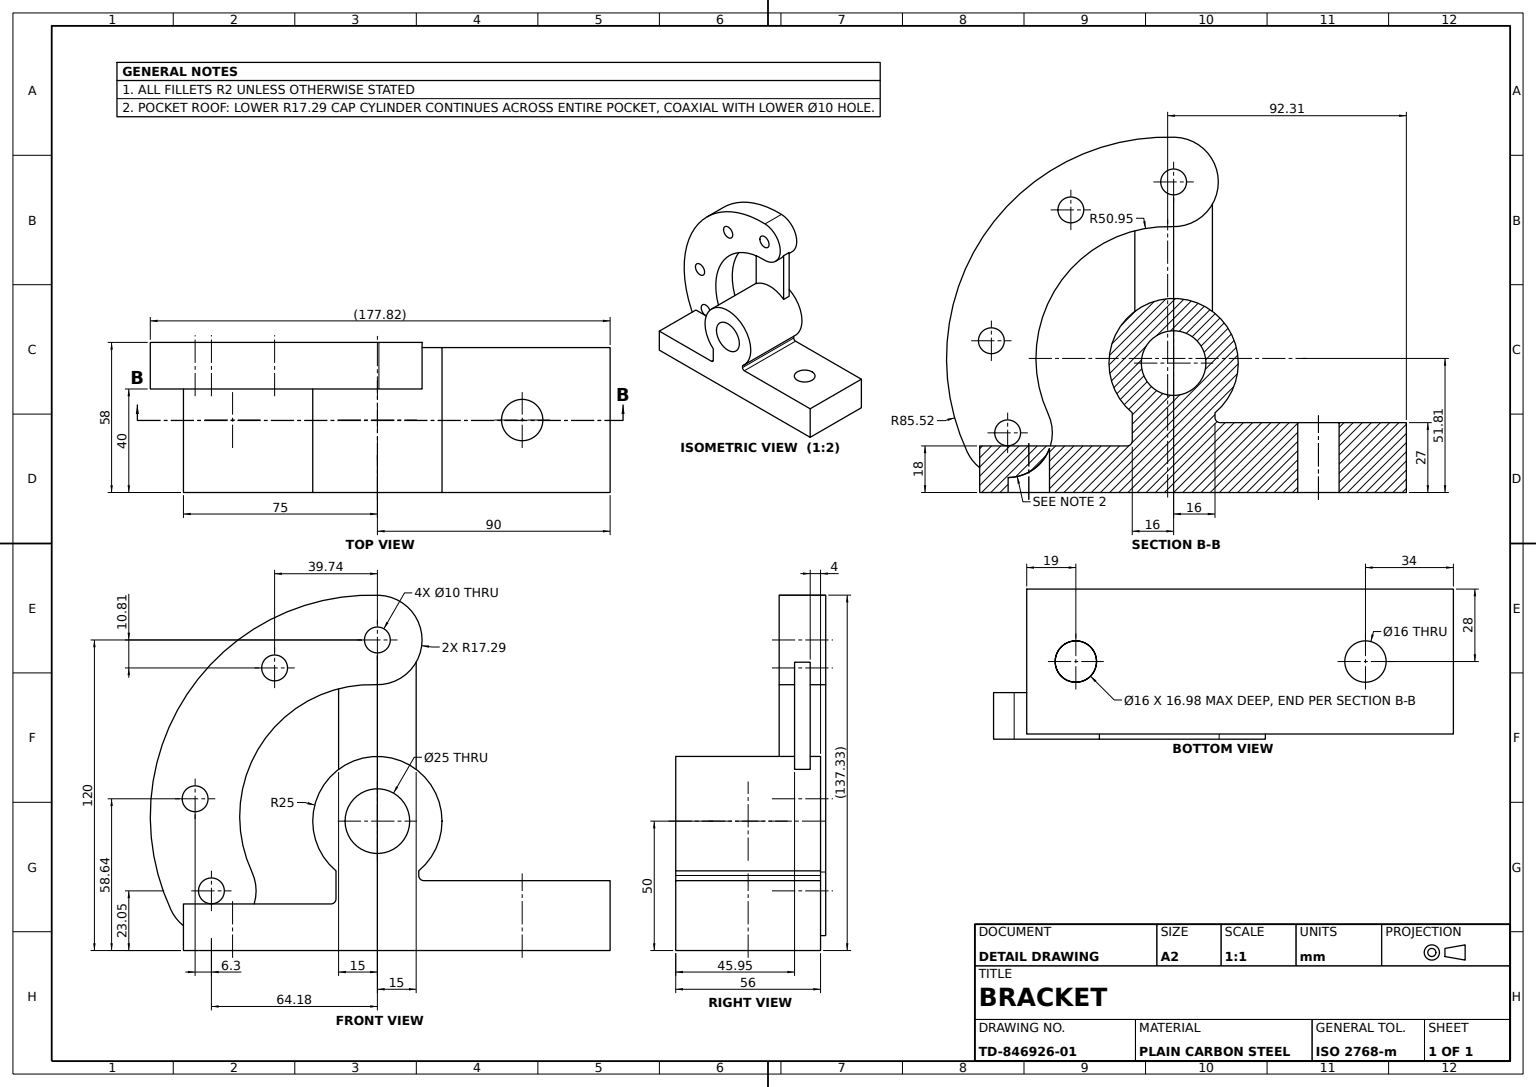
ISO-10303-21;
HEADER;
FILE_DESCRIPTION((''),'2;1');
FILE_NAME('','',(''),(''),'','','');
FILE_SCHEMA(('AUTOMOTIVE_DESIGN'));
ENDSEC;
DATA;
#1=APPLICATION_CONTEXT('');
#2=PRODUCT_CONTEXT('',#1,'mechanical');
#3=PRODUCT('','','',(#2));
#4=PRODUCT_DEFINITION_FORMATION('','',#3);
#5=PRODUCT_DEFINITION_CONTEXT('',#1,'design');
#6=PRODUCT_DEFINITION('','',#4,#5);
#7=PRODUCT_DEFINITION_SHAPE('','',#6);
#8=(LENGTH_UNIT()NAMED_UNIT(*)SI_UNIT(.MILLI.,.METRE.));
#9=(NAMED_UNIT(*)PLANE_ANGLE_UNIT()SI_UNIT($,.RADIAN.));
#10=(NAMED_UNIT(*)SI_UNIT($,.STERADIAN.)SOLID_ANGLE_UNIT());
#11=UNCERTAINTY_MEASURE_WITH_UNIT(LENGTH_MEASURE(1.E-05),#8,'distance_accuracy_value','');
#12=(GEOMETRIC_REPRESENTATION_CONTEXT(3)GLOBAL_UNCERTAINTY_ASSIGNED_CONTEXT((#11))GLOBAL_UNIT_ASSIGNED_CONTEXT((#8,#9,#10))REPRESENTATION_CONTEXT('',''));
#13=CARTESIAN_POINT('',(-5.,120.,-40.));
#14=VERTEX_POINT('',#13);
#15=CARTESIAN_POINT('',(-5.,120.,-58.));
#16=VERTEX_POINT('',#15);
#17=CARTESIAN_POINT('',(-5.,120.,-18.));
#18=DIRECTION('',(0.,0.,-1.));
#19=VECTOR('',#18,1000.);
#20=LINE('',#17,#19);
#21=EDGE_CURVE('',#14,#16,#20,.T.);
#22=ORIENTED_EDGE('',*,*,#21,.T.);
#23=CARTESIAN_POINT('',(5.,120.,-58.));
#24=VERTEX_POINT('',#23);
#25=CARTESIAN_POINT('',(0.,120.,-58.));
#26=DIRECTION('',(-1.,0.,0.));
#27=AXIS2_PLACEMENT_3D('',#25,#18,#26);
#28=CIRCLE('',#27,5.);
#29=EDGE_CURVE('',#16,#24,#28,.T.);
#30=ORIENTED_EDGE('',*,*,#29,.T.);
#31=CARTESIAN_POINT('',(5.,120.,-40.));
#32=VERTEX_POINT('',#31);
#33=CARTESIAN_POINT('',(5.,120.,-18.));
#34=LINE('',#33,#19);
#35=EDGE_CURVE('',#32,#24,#34,.T.);
#36=ORIENTED_EDGE('',*,*,#35,.F.);
#37=CARTESIAN_POINT('',(0.,120.,-40.));
#38=DIRECTION('',(0.,0.,1.));
#39=DIRECTION('',(1.,0.,0.));
#40=AXIS2_PLACEMENT_3D('',#37,#38,#39);
#41=CIRCLE('',#40,5.);
#42=EDGE_CURVE('',#32,#14,#41,.T.);
#43=ORIENTED_EDGE('',*,*,#42,.T.);
#44=EDGE_LOOP('',(#22,#30,#36,#43));
#45=FACE_OUTER_BOUND('',#44,.T.);
#46=CARTESIAN_POINT('',(0.,120.,-18.));
#47=AXIS2_PLACEMENT_3D('',#46,#18,#26);
#48=CYLINDRICAL_SURFACE('',#47,5.);
#49=ADVANCED_FACE('',(#45),#48,.F.);
#50=CARTESIAN_POINT('',(-12.5,50.,-56.));
#51=VERTEX_POINT('',#50);
#52=CARTESIAN_POINT('',(-12.5,50.,0.));
#53=VERTEX_POINT('',#52);
#54=VECTOR('',#38,1000.);
#55=LINE('',#50,#54);
#56=EDGE_CURVE('',#51,#53,#55,.T.);
#57=ORIENTED_EDGE('',*,*,#56,.T.);
#58=CARTESIAN_POINT('',(12.5,50.,0.));
#59=VERTEX_POINT('',#58);
#60=CARTESIAN_POINT('',(0.,50.,0.));
#61=AXIS2_PLACEMENT_3D('',#60,#38,#39);
#62=CIRCLE('',#61,12.5);
#63=EDGE_CURVE('',#53,#59,#62,.T.);
#64=ORIENTED_EDGE('',*,*,#63,.T.);
#65=CARTESIAN_POINT('',(12.5,50.,-56.));
#66=VERTEX_POINT('',#65);
#67=LINE('',#65,#54);
#68=EDGE_CURVE('',#66,#59,#67,.T.);
#69=ORIENTED_EDGE('',*,*,#68,.F.);
#70=CARTESIAN_POINT('',(0.,50.,-56.));
#71=AXIS2_PLACEMENT_3D('',#70,#38,#39);
#72=CIRCLE('',#71,12.5);
#73=EDGE_CURVE('',#51,#66,#72,.T.);
#74=ORIENTED_EDGE('',*,*,#73,.F.);
#75=EDGE_LOOP('',(#57,#64,#69,#74));
#76=FACE_OUTER_BOUND('',#75,.T.);
#77=CYLINDRICAL_SURFACE('',#71,12.5);
#78=ADVANCED_FACE('',(#76),#77,.F.);
#79=CARTESIAN_POINT('',(-69.182521,23.053551,-40.));
#80=VERTEX_POINT('',#79);
#81=CARTESIAN_POINT('',(-59.182521,23.053551,-40.));
#82=VERTEX_POINT('',#81);
#83=CARTESIAN_POINT('',(-64.182521,23.053551,-40.));
#84=AXIS2_PLACEMENT_3D('',#83,#38,#39);
#85=CIRCLE('',#84,5.);
#86=EDGE_CURVE('',#80,#82,#85,.T.);
#87=ORIENTED_EDGE('',*,*,#86,.T.);
#88=CARTESIAN_POINT('',(-59.182521,23.053551,-58.));
#89=VERTEX_POINT('',#88);
#90=CARTESIAN_POINT('',(-59.182521,23.053551,-18.));
#91=LINE('',#90,#19);
#92=EDGE_CURVE('',#82,#89,#91,.T.);
#93=ORIENTED_EDGE('',*,*,#92,.T.);
#94=CARTESIAN_POINT('',(-69.182521,23.053551,-58.));
#95=VERTEX_POINT('',#94);
#96=CARTESIAN_POINT('',(-64.182521,23.053551,-58.));
#97=AXIS2_PLACEMENT_3D('',#96,#18,#26);
#98=CIRCLE('',#97,5.);
#99=EDGE_CURVE('',#89,#95,#98,.T.);
#100=ORIENTED_EDGE('',*,*,#99,.T.);
#101=CARTESIAN_POINT('',(-69.182521,23.053551,-18.));
#102=LINE('',#101,#19);
#103=EDGE_CURVE('',#80,#95,#102,.T.);
#104=ORIENTED_EDGE('',*,*,#103,.F.);
#105=EDGE_LOOP('',(#87,#93,#100,#104));
#106=FACE_OUTER_BOUND('',#105,.T.);
#107=CARTESIAN_POINT('',(-64.182521,23.053551,-18.));
#108=AXIS2_PLACEMENT_3D('',#107,#18,#26);
#109=CYLINDRICAL_SURFACE('',#108,5.);
#110=ADVANCED_FACE('',(#106),#109,.F.);
#111=CARTESIAN_POINT('',(15.,111.408742,-45.952641));
#112=VERTEX_POINT('',#111);
#113=CARTESIAN_POINT('',(15.,111.408742,-52.));
#114=VERTEX_POINT('',#113);
#115=CARTESIAN_POINT('',(15.,111.408742,-58.));
#116=LINE('',#115,#19);
#117=EDGE_CURVE('',#112,#114,#116,.T.);
#118=ORIENTED_EDGE('',*,*,#117,.F.);
#119=CARTESIAN_POINT('',(15.,70.,-45.952641));
#120=VERTEX_POINT('',#119);
#121=CARTESIAN_POINT('',(15.,-0.001,-45.952641));
#122=DIRECTION('',(0.,1.,0.));
#123=VECTOR('',#122,1000.);
#124=LINE('',#121,#123);
#125=EDGE_CURVE('',#120,#112,#124,.T.);
#126=ORIENTED_EDGE('',*,*,#125,.F.);
#127=CARTESIAN_POINT('',(15.,70.,-52.));
#128=VERTEX_POINT('',#127);
#129=CARTESIAN_POINT('',(15.,70.,-56.));
#130=LINE('',#129,#19);
#131=EDGE_CURVE('',#120,#128,#130,.T.);
#132=ORIENTED_EDGE('',*,*,#131,.T.);
#133=CARTESIAN_POINT('',(15.,65.595641,-52.));
#134=LINE('',#133,#123);
#135=EDGE_CURVE('',#128,#114,#134,.T.);
#136=ORIENTED_EDGE('',*,*,#135,.T.);
#137=EDGE_LOOP('',(#118,#126,#132,#136));
#138=FACE_OUTER_BOUND('',#137,.T.);
#139=CARTESIAN_POINT('',(15.,65.595641,-118.127564));
#140=AXIS2_PLACEMENT_3D('',#139,#39,#18);
#141=PLANE('',#140);
#142=ADVANCED_FACE('',(#138),#141,.T.);
#143=CARTESIAN_POINT('',(56.,0.,-20.));
#144=VERTEX_POINT('',#143);
#145=CARTESIAN_POINT('',(56.,0.,-36.));
#146=VERTEX_POINT('',#145);
#147=CARTESIAN_POINT('',(56.,0.,-28.));
#148=AXIS2_PLACEMENT_3D('',#147,#122,#38);
#149=CIRCLE('',#148,8.);
#150=EDGE_CURVE('',#144,#146,#149,.T.);
#151=ORIENTED_EDGE('',*,*,#150,.T.);
#152=EDGE_CURVE('',#146,#144,#149,.T.);
#153=ORIENTED_EDGE('',*,*,#152,.T.);
#154=EDGE_LOOP('',(#151,#153));
#155=FACE_BOUND('',#154,.T.);
#156=CARTESIAN_POINT('',(-56.,0.,-20.));
#157=VERTEX_POINT('',#156);
#158=CARTESIAN_POINT('',(-56.,0.,-36.));
#159=VERTEX_POINT('',#158);
#160=CARTESIAN_POINT('',(-56.,0.,-28.));
#161=AXIS2_PLACEMENT_3D('',#160,#122,#18);
#162=CIRCLE('',#161,8.);
#163=EDGE_CURVE('',#157,#159,#162,.T.);
#164=ORIENTED_EDGE('',*,*,#163,.T.);
#165=EDGE_CURVE('',#159,#157,#162,.T.);
#166=ORIENTED_EDGE('',*,*,#165,.T.);
#167=EDGE_LOOP('',(#164,#166));
#168=FACE_BOUND('',#167,.T.);
#169=CARTESIAN_POINT('',(90.,0.,-56.));
#170=VERTEX_POINT('',#169);
#171=CARTESIAN_POINT('',(90.,0.,0.));
#172=VERTEX_POINT('',#171);
#173=LINE('',#169,#54);
#174=EDGE_CURVE('',#170,#172,#173,.T.);
#175=ORIENTED_EDGE('',*,*,#174,.T.);
#176=CARTESIAN_POINT('',(-75.,0.,0.));
#177=VERTEX_POINT('',#176);
#178=CARTESIAN_POINT('',(0.,0.,0.));
#179=VECTOR('',#39,1000.);
#180=LINE('',#178,#179);
#181=EDGE_CURVE('',#177,#172,#180,.T.);
#182=ORIENTED_EDGE('',*,*,#181,.F.);
#183=CARTESIAN_POINT('',(-75.,0.,-56.));
#184=VERTEX_POINT('',#183);
#185=LINE('',#183,#54);
#186=EDGE_CURVE('',#184,#177,#185,.T.);
#187=ORIENTED_EDGE('',*,*,#186,.F.);
#188=LINE('',#169,#179);
#189=EDGE_CURVE('',#184,#170,#188,.T.);
#190=ORIENTED_EDGE('',*,*,#189,.T.);
#191=EDGE_LOOP('',(#175,#182,#187,#190));
#192=FACE_OUTER_BOUND('',#191,.T.);
#193=CARTESIAN_POINT('',(0.,0.,-56.));
#194=DIRECTION('',(0.,-1.,0.));
#195=AXIS2_PLACEMENT_3D('',#193,#194,#18);
#196=PLANE('',#195);
#197=ADVANCED_FACE('',(#155,#168,#192),#196,.T.);
#198=CARTESIAN_POINT('',(56.,27.,-36.));
#199=VERTEX_POINT('',#198);
#200=LINE('',#145,#123);
#201=EDGE_CURVE('',#146,#199,#200,.T.);
#202=ORIENTED_EDGE('',*,*,#201,.T.);
#203=CARTESIAN_POINT('',(56.,27.,-20.));
#204=VERTEX_POINT('',#203);
#205=CARTESIAN_POINT('',(56.,27.,-28.));
#206=AXIS2_PLACEMENT_3D('',#205,#122,#38);
#207=CIRCLE('',#206,8.);
#208=EDGE_CURVE('',#199,#204,#207,.T.);
#209=ORIENTED_EDGE('',*,*,#208,.T.);
#210=LINE('',#143,#123);
#211=EDGE_CURVE('',#144,#204,#210,.T.);
#212=ORIENTED_EDGE('',*,*,#211,.F.);
#213=ORIENTED_EDGE('',*,*,#152,.F.);
#214=EDGE_LOOP('',(#202,#209,#212,#213));
#215=FACE_OUTER_BOUND('',#214,.T.);
#216=CYLINDRICAL_SURFACE('',#148,8.);
#217=ADVANCED_FACE('',(#215),#216,.F.);
#218=CARTESIAN_POINT('',(-16.,30.790627,-56.));
#219=VERTEX_POINT('',#218);
#220=CARTESIAN_POINT('',(-16.,20.,-56.));
#221=VERTEX_POINT('',#220);
#222=VECTOR('',#194,1000.);
#223=LINE('',#218,#222);
#224=EDGE_CURVE('',#219,#221,#223,.T.);
#225=ORIENTED_EDGE('',*,*,#224,.T.);
#226=CARTESIAN_POINT('',(-16.,20.,0.));
#227=VERTEX_POINT('',#226);
#228=LINE('',#226,#54);
#229=EDGE_CURVE('',#221,#227,#228,.T.);
#230=ORIENTED_EDGE('',*,*,#229,.T.);
#231=CARTESIAN_POINT('',(-16.,30.790627,0.));
#232=VERTEX_POINT('',#231);
#233=LINE('',#231,#222);
#234=EDGE_CURVE('',#232,#227,#233,.T.);
#235=ORIENTED_EDGE('',*,*,#234,.F.);
#236=LINE('',#218,#54);
#237=EDGE_CURVE('',#219,#232,#236,.T.);
#238=ORIENTED_EDGE('',*,*,#237,.F.);
#239=EDGE_LOOP('',(#225,#230,#235,#238));
#240=FACE_OUTER_BOUND('',#239,.T.);
#241=AXIS2_PLACEMENT_3D('',#218,#26,#194);
#242=PLANE('',#241);
#243=ADVANCED_FACE('',(#240),#242,.T.);
#244=CARTESIAN_POINT('',(-25.,50.,-56.));
#245=VERTEX_POINT('',#244);
#246=CARTESIAN_POINT('',(-25.,50.,0.));
#247=VERTEX_POINT('',#246);
#248=LINE('',#244,#54);
#249=EDGE_CURVE('',#245,#247,#248,.T.);
#250=ORIENTED_EDGE('',*,*,#249,.F.);
#251=CIRCLE('',#71,25.);
#252=EDGE_CURVE('',#245,#219,#251,.T.);
#253=ORIENTED_EDGE('',*,*,#252,.T.);
#254=ORIENTED_EDGE('',*,*,#237,.T.);
#255=CIRCLE('',#61,25.);
#256=EDGE_CURVE('',#247,#232,#255,.T.);
#257=ORIENTED_EDGE('',*,*,#256,.F.);
#258=EDGE_LOOP('',(#250,#253,#254,#257));
#259=FACE_OUTER_BOUND('',#258,.T.);
#260=CYLINDRICAL_SURFACE('',#71,25.);
#261=ADVANCED_FACE('',(#259),#260,.T.);
#262=ORIENTED_EDGE('',*,*,#63,.F.);
#263=EDGE_CURVE('',#59,#53,#62,.T.);
#264=ORIENTED_EDGE('',*,*,#263,.F.);
#265=EDGE_LOOP('',(#262,#264));
#266=FACE_BOUND('',#265,.T.);
#267=CARTESIAN_POINT('',(90.,27.,0.));
#268=VERTEX_POINT('',#267);
#269=CARTESIAN_POINT('',(18.,27.,0.));
#270=VERTEX_POINT('',#269);
#271=CARTESIAN_POINT('',(0.,27.,0.));
#272=VECTOR('',#26,1000.);
#273=LINE('',#271,#272);
#274=EDGE_CURVE('',#268,#270,#273,.T.);
#275=ORIENTED_EDGE('',*,*,#274,.T.);
#276=CARTESIAN_POINT('',(16.,29.,0.));
#277=VERTEX_POINT('',#276);
#278=CARTESIAN_POINT('',(18.,29.,0.));
#279=AXIS2_PLACEMENT_3D('',#278,#18,#26);
#280=CIRCLE('',#279,2.);
#281=EDGE_CURVE('',#270,#277,#280,.T.);
#282=ORIENTED_EDGE('',*,*,#281,.T.);
#283=CARTESIAN_POINT('',(16.,30.790627,0.));
#284=VERTEX_POINT('',#283);
#285=LINE('',#283,#123);
#286=EDGE_CURVE('',#277,#284,#285,.T.);
#287=ORIENTED_EDGE('',*,*,#286,.T.);
#288=CARTESIAN_POINT('',(25.,50.,0.));
#289=VERTEX_POINT('',#288);
#290=EDGE_CURVE('',#284,#289,#255,.T.);
#291=ORIENTED_EDGE('',*,*,#290,.T.);
#292=EDGE_CURVE('',#289,#247,#255,.T.);
#293=ORIENTED_EDGE('',*,*,#292,.T.);
#294=ORIENTED_EDGE('',*,*,#256,.T.);
#295=ORIENTED_EDGE('',*,*,#234,.T.);
#296=CARTESIAN_POINT('',(-18.,18.,0.));
#297=VERTEX_POINT('',#296);
#298=CARTESIAN_POINT('',(-18.,20.,0.));
#299=AXIS2_PLACEMENT_3D('',#298,#18,#26);
#300=CIRCLE('',#299,2.);
#301=EDGE_CURVE('',#227,#297,#300,.T.);
#302=ORIENTED_EDGE('',*,*,#301,.T.);
#303=CARTESIAN_POINT('',(-75.,18.,0.));
#304=VERTEX_POINT('',#303);
#305=LINE('',#303,#272);
#306=EDGE_CURVE('',#297,#304,#305,.T.);
#307=ORIENTED_EDGE('',*,*,#306,.T.);
#308=LINE('',#176,#222);
#309=EDGE_CURVE('',#304,#177,#308,.T.);
#310=ORIENTED_EDGE('',*,*,#309,.T.);
#311=ORIENTED_EDGE('',*,*,#181,.T.);
#312=LINE('',#267,#123);
#313=EDGE_CURVE('',#172,#268,#312,.T.);
#314=ORIENTED_EDGE('',*,*,#313,.T.);
#315=EDGE_LOOP('',(#275,#282,#287,#291,#293,#294,#295,#302,#307,#310,#311,#314));
#316=FACE_OUTER_BOUND('',#315,.T.);
#317=AXIS2_PLACEMENT_3D('',#178,#18,#26);
#318=PLANE('',#317);
#319=ADVANCED_FACE('',(#266,#316),#318,.F.);
#320=ORIENTED_EDGE('',*,*,#286,.F.);
#321=CARTESIAN_POINT('',(16.,29.,-56.));
#322=VERTEX_POINT('',#321);
#323=LINE('',#321,#19);
#324=EDGE_CURVE('',#277,#322,#323,.T.);
#325=ORIENTED_EDGE('',*,*,#324,.T.);
#326=CARTESIAN_POINT('',(16.,30.790627,-56.));
#327=VERTEX_POINT('',#326);
#328=LINE('',#326,#123);
#329=EDGE_CURVE('',#322,#327,#328,.T.);
#330=ORIENTED_EDGE('',*,*,#329,.T.);
#331=LINE('',#326,#54);
#332=EDGE_CURVE('',#327,#284,#331,.T.);
#333=ORIENTED_EDGE('',*,*,#332,.T.);
#334=EDGE_LOOP('',(#320,#325,#330,#333));
#335=FACE_OUTER_BOUND('',#334,.T.);
#336=AXIS2_PLACEMENT_3D('',#326,#39,#122);
#337=PLANE('',#336);
#338=ADVANCED_FACE('',(#335),#337,.T.);
#339=ORIENTED_EDGE('',*,*,#281,.F.);
#340=CARTESIAN_POINT('',(18.,27.,-56.));
#341=VERTEX_POINT('',#340);
#342=LINE('',#269,#54);
#343=EDGE_CURVE('',#341,#270,#342,.T.);
#344=ORIENTED_EDGE('',*,*,#343,.F.);
#345=CARTESIAN_POINT('',(18.,29.,-56.));
#346=AXIS2_PLACEMENT_3D('',#345,#38,#26);
#347=CIRCLE('',#346,2.);
#348=EDGE_CURVE('',#322,#341,#347,.T.);
#349=ORIENTED_EDGE('',*,*,#348,.F.);
#350=ORIENTED_EDGE('',*,*,#324,.F.);
#351=EDGE_LOOP('',(#339,#344,#349,#350));
#352=FACE_OUTER_BOUND('',#351,.T.);
#353=AXIS2_PLACEMENT_3D('',#345,#38,#39);
#354=CYLINDRICAL_SURFACE('',#353,2.);
#355=ADVANCED_FACE('',(#352),#354,.F.);
#356=CARTESIAN_POINT('',(-79.858671,15.768771,-58.));
#357=VERTEX_POINT('',#356);
#358=CARTESIAN_POINT('',(-79.858671,15.768771,-40.));
#359=VERTEX_POINT('',#358);
#360=LINE('',#356,#54);
#361=EDGE_CURVE('',#357,#359,#360,.T.);
#362=ORIENTED_EDGE('',*,*,#361,.F.);
#363=CARTESIAN_POINT('',(-46.896408,23.053551,-58.));
#364=VERTEX_POINT('',#363);
#365=AXIS2_PLACEMENT_3D('',#96,#38,#39);
#366=CIRCLE('',#365,17.286113);
#367=EDGE_CURVE('',#357,#364,#366,.T.);
#368=ORIENTED_EDGE('',*,*,#367,.T.);
#369=CARTESIAN_POINT('',(-46.896408,23.053551,-40.));
#370=VERTEX_POINT('',#369);
#371=LINE('',#363,#54);
#372=EDGE_CURVE('',#364,#370,#371,.T.);
#373=ORIENTED_EDGE('',*,*,#372,.T.);
#374=CARTESIAN_POINT('',(-47.651601,18.,-40.));
#375=VERTEX_POINT('',#374);
#376=CIRCLE('',#84,17.286113);
#377=EDGE_CURVE('',#375,#370,#376,.T.);
#378=ORIENTED_EDGE('',*,*,#377,.F.);
#379=CARTESIAN_POINT('',(-47.651601,18.,-56.));
#380=VERTEX_POINT('',#379);
#381=CARTESIAN_POINT('',(-47.651601,18.,-58.));
#382=LINE('',#381,#19);
#383=EDGE_CURVE('',#375,#380,#382,.T.);
#384=ORIENTED_EDGE('',*,*,#383,.T.);
#385=CARTESIAN_POINT('',(-75.,9.57053,-56.));
#386=VERTEX_POINT('',#385);
#387=CARTESIAN_POINT('',(-64.182521,23.053551,-56.));
#388=AXIS2_PLACEMENT_3D('',#387,#18,#26);
#389=CIRCLE('',#388,17.286113);
#390=EDGE_CURVE('',#380,#386,#389,.T.);
#391=ORIENTED_EDGE('',*,*,#390,.T.);
#392=CARTESIAN_POINT('',(-75.,9.57053,-40.));
#393=VERTEX_POINT('',#392);
#394=CARTESIAN_POINT('',(-75.,9.57053,-58.));
#395=LINE('',#394,#54);
#396=EDGE_CURVE('',#386,#393,#395,.T.);
#397=ORIENTED_EDGE('',*,*,#396,.T.);
#398=EDGE_CURVE('',#359,#393,#376,.T.);
#399=ORIENTED_EDGE('',*,*,#398,.F.);
#400=EDGE_LOOP('',(#362,#368,#373,#378,#384,#391,#397,#399));
#401=FACE_OUTER_BOUND('',#400,.T.);
#402=CYLINDRICAL_SURFACE('',#365,17.286113);
#403=ADVANCED_FACE('',(#401),#402,.T.);
#404=CARTESIAN_POINT('',(-75.482391,58.635503,-40.));
#405=VERTEX_POINT('',#404);
#406=CARTESIAN_POINT('',(-75.482391,58.635503,-58.));
#407=VERTEX_POINT('',#406);
#408=CARTESIAN_POINT('',(-75.482391,58.635503,-18.));
#409=LINE('',#408,#19);
#410=EDGE_CURVE('',#405,#407,#409,.T.);
#411=ORIENTED_EDGE('',*,*,#410,.F.);
#412=CARTESIAN_POINT('',(-65.482391,58.635503,-40.));
#413=VERTEX_POINT('',#412);
#414=CARTESIAN_POINT('',(-70.482391,58.635503,-40.));
#415=AXIS2_PLACEMENT_3D('',#414,#38,#39);
#416=CIRCLE('',#415,5.);
#417=EDGE_CURVE('',#405,#413,#416,.T.);
#418=ORIENTED_EDGE('',*,*,#417,.T.);
#419=CARTESIAN_POINT('',(-65.482391,58.635503,-58.));
#420=VERTEX_POINT('',#419);
#421=CARTESIAN_POINT('',(-65.482391,58.635503,-18.));
#422=LINE('',#421,#19);
#423=EDGE_CURVE('',#413,#420,#422,.T.);
#424=ORIENTED_EDGE('',*,*,#423,.T.);
#425=CARTESIAN_POINT('',(-70.482391,58.635503,-58.));
#426=AXIS2_PLACEMENT_3D('',#425,#18,#26);
#427=CIRCLE('',#426,5.);
#428=EDGE_CURVE('',#420,#407,#427,.T.);
#429=ORIENTED_EDGE('',*,*,#428,.T.);
#430=EDGE_LOOP('',(#411,#418,#424,#429));
#431=FACE_OUTER_BOUND('',#430,.T.);
#432=CARTESIAN_POINT('',(-70.482391,58.635503,-18.));
#433=AXIS2_PLACEMENT_3D('',#432,#18,#26);
#434=CYLINDRICAL_SURFACE('',#433,5.);
#435=ADVANCED_FACE('',(#431),#434,.F.);
#436=ORIENTED_EDGE('',*,*,#417,.F.);
#437=EDGE_CURVE('',#413,#405,#416,.T.);
#438=ORIENTED_EDGE('',*,*,#437,.F.);
#439=EDGE_LOOP('',(#436,#438));
#440=FACE_BOUND('',#439,.T.);
#441=ORIENTED_EDGE('',*,*,#86,.F.);
#442=EDGE_CURVE('',#82,#80,#85,.T.);
#443=ORIENTED_EDGE('',*,*,#442,.F.);
#444=EDGE_LOOP('',(#441,#443));
#445=FACE_BOUND('',#444,.T.);
#446=EDGE_CURVE('',#14,#32,#41,.T.);
#447=ORIENTED_EDGE('',*,*,#446,.F.);
#448=ORIENTED_EDGE('',*,*,#42,.F.);
#449=EDGE_LOOP('',(#447,#448));
#450=FACE_BOUND('',#449,.T.);
#451=CARTESIAN_POINT('',(17.286113,120.,-40.));
#452=VERTEX_POINT('',#451);
#453=CARTESIAN_POINT('',(0.584249,137.276237,-40.));
#454=VERTEX_POINT('',#453);
#455=CIRCLE('',#40,17.286113);
#456=EDGE_CURVE('',#452,#454,#455,.T.);
#457=ORIENTED_EDGE('',*,*,#456,.T.);
#458=CARTESIAN_POINT('',(-2.30613,51.807799,-40.));
#459=AXIS2_PLACEMENT_3D('',#458,#38,#39);
#460=CIRCLE('',#459,85.517298);
#461=EDGE_CURVE('',#454,#359,#460,.T.);
#462=ORIENTED_EDGE('',*,*,#461,.T.);
#463=ORIENTED_EDGE('',*,*,#398,.T.);
#464=CARTESIAN_POINT('',(-75.,18.,-40.));
#465=VERTEX_POINT('',#464);
#466=LINE('',#464,#123);
#467=EDGE_CURVE('',#393,#465,#466,.T.);
#468=ORIENTED_EDGE('',*,*,#467,.T.);
#469=LINE('',#374,#179);
#470=EDGE_CURVE('',#465,#375,#469,.T.);
#471=ORIENTED_EDGE('',*,*,#470,.T.);
#472=ORIENTED_EDGE('',*,*,#377,.T.);
#473=CARTESIAN_POINT('',(-48.506371,30.338332,-40.));
#474=VERTEX_POINT('',#473);
#475=EDGE_CURVE('',#370,#474,#376,.T.);
#476=ORIENTED_EDGE('',*,*,#475,.T.);
#477=CARTESIAN_POINT('',(-0.584249,102.723763,-40.));
#478=VERTEX_POINT('',#477);
#479=CIRCLE('',#459,50.945071);
#480=EDGE_CURVE('',#478,#474,#479,.T.);
#481=ORIENTED_EDGE('',*,*,#480,.F.);
#482=EDGE_CURVE('',#478,#452,#455,.T.);
#483=ORIENTED_EDGE('',*,*,#482,.T.);
#484=EDGE_LOOP('',(#457,#462,#463,#468,#471,#472,#476,#481,#483));
#485=FACE_OUTER_BOUND('',#484,.T.);
#486=CARTESIAN_POINT('',(-44.743103,109.193277,-40.));
#487=VERTEX_POINT('',#486);
#488=CARTESIAN_POINT('',(-34.743103,109.193277,-40.));
#489=VERTEX_POINT('',#488);
#490=CARTESIAN_POINT('',(-39.743103,109.193277,-40.));
#491=AXIS2_PLACEMENT_3D('',#490,#38,#39);
#492=CIRCLE('',#491,5.);
#493=EDGE_CURVE('',#487,#489,#492,.T.);
#494=ORIENTED_EDGE('',*,*,#493,.F.);
#495=EDGE_CURVE('',#489,#487,#492,.T.);
#496=ORIENTED_EDGE('',*,*,#495,.F.);
#497=EDGE_LOOP('',(#494,#496));
#498=FACE_BOUND('',#497,.T.);
#499=CARTESIAN_POINT('',(-1.153065,85.903899,-40.));
#500=AXIS2_PLACEMENT_3D('',#499,#38,#39);
#501=PLANE('',#500);
#502=ADVANCED_FACE('',(#440,#445,#450,#485,#498),#501,.T.);
#503=EDGE_CURVE('',#407,#420,#427,.T.);
#504=ORIENTED_EDGE('',*,*,#503,.T.);
#505=ORIENTED_EDGE('',*,*,#423,.F.);
#506=ORIENTED_EDGE('',*,*,#437,.T.);
#507=ORIENTED_EDGE('',*,*,#410,.T.);
#508=EDGE_LOOP('',(#504,#505,#506,#507));
#509=FACE_OUTER_BOUND('',#508,.T.);
#510=ADVANCED_FACE('',(#509),#434,.F.);
#511=CARTESIAN_POINT('',(-15.,70.,-52.));
#512=VERTEX_POINT('',#511);
#513=CARTESIAN_POINT('',(0.,50.,-52.));
#514=AXIS2_PLACEMENT_3D('',#513,#38,#26);
#515=CIRCLE('',#514,25.);
#516=EDGE_CURVE('',#128,#512,#515,.T.);
#517=ORIENTED_EDGE('',*,*,#516,.T.);
#518=CARTESIAN_POINT('',(-15.,101.14608,-52.));
#519=VERTEX_POINT('',#518);
#520=CARTESIAN_POINT('',(-15.,65.595641,-52.));
#521=LINE('',#520,#123);
#522=EDGE_CURVE('',#512,#519,#521,.T.);
#523=ORIENTED_EDGE('',*,*,#522,.T.);
#524=CARTESIAN_POINT('',(-0.584249,102.723763,-52.));
#525=VERTEX_POINT('',#524);
#526=CARTESIAN_POINT('',(-2.30613,51.807799,-52.));
#527=AXIS2_PLACEMENT_3D('',#526,#38,#26);
#528=CIRCLE('',#527,50.945071);
#529=EDGE_CURVE('',#525,#519,#528,.T.);
#530=ORIENTED_EDGE('',*,*,#529,.F.);
#531=CARTESIAN_POINT('',(0.,120.,-52.));
#532=AXIS2_PLACEMENT_3D('',#531,#18,#26);
#533=CIRCLE('',#532,17.286113);
#534=EDGE_CURVE('',#114,#525,#533,.T.);
#535=ORIENTED_EDGE('',*,*,#534,.F.);
#536=ORIENTED_EDGE('',*,*,#135,.F.);
#537=EDGE_LOOP('',(#517,#523,#530,#535,#536));
#538=FACE_OUTER_BOUND('',#537,.T.);
#539=CARTESIAN_POINT('',(0.,0.,-52.));
#540=AXIS2_PLACEMENT_3D('',#539,#18,#26);
#541=PLANE('',#540);
#542=ADVANCED_FACE('',(#538),#541,.T.);
#543=ORIENTED_EDGE('',*,*,#211,.T.);
#544=EDGE_CURVE('',#204,#199,#207,.T.);
#545=ORIENTED_EDGE('',*,*,#544,.T.);
#546=ORIENTED_EDGE('',*,*,#201,.F.);
#547=ORIENTED_EDGE('',*,*,#150,.F.);
#548=EDGE_LOOP('',(#543,#545,#546,#547));
#549=FACE_OUTER_BOUND('',#548,.T.);
#550=ADVANCED_FACE('',(#549),#216,.F.);
#551=CARTESIAN_POINT('',(-56.,7.826731,-36.));
#552=VERTEX_POINT('',#551);
#553=CARTESIAN_POINT('',(-56.,7.826731,-20.));
#554=VERTEX_POINT('',#553);
#555=CARTESIAN_POINT('',(-55.711029,7.982017,-36.));
#556=CARTESIAN_POINT('',(-55.423806,8.147112,-35.984164));
#557=CARTESIAN_POINT('',(-54.865332,8.489657,-35.924103));
#558=CARTESIAN_POINT('',(-54.593559,8.66726,-35.880053));
#559=CARTESIAN_POINT('',(-54.063978,9.034684,-35.766925));
#560=CARTESIAN_POINT('',(-53.806172,9.224506,-35.697837));
#561=CARTESIAN_POINT('',(-53.303879,9.616057,-35.536611));
#562=CARTESIAN_POINT('',(-53.058655,9.8185,-35.444065));
#563=CARTESIAN_POINT('',(-52.353331,10.433365,-35.138928));
#564=CARTESIAN_POINT('',(-51.919837,10.855781,-34.898414));
#565=CARTESIAN_POINT('',(-51.115333,11.721842,-34.354202));
#566=CARTESIAN_POINT('',(-50.744413,12.165561,-34.05048));
#567=CARTESIAN_POINT('',(-50.059912,13.069415,-33.380043));
#568=CARTESIAN_POINT('',(-49.753172,13.520583,-33.020246));
#569=CARTESIAN_POINT('',(-49.202895,14.41096,-32.245595));
#570=CARTESIAN_POINT('',(-48.959248,14.85088,-31.831537));
#571=CARTESIAN_POINT('',(-48.64098,15.482175,-31.147703));
#572=CARTESIAN_POINT('',(-48.542359,15.688747,-30.907627));
#573=CARTESIAN_POINT('',(-48.365751,16.076101,-30.406023));
#574=CARTESIAN_POINT('',(-48.287443,16.25749,-30.144394));
#575=CARTESIAN_POINT('',(-48.153886,16.578767,-29.587598));
#576=CARTESIAN_POINT('',(-48.098155,16.719977,-29.288226));
#577=CARTESIAN_POINT('',(-48.040641,16.868713,-28.82053));
#578=CARTESIAN_POINT('',(-48.025693,16.90803,-28.661227));
#579=CARTESIAN_POINT('',(-48.005319,16.961863,-28.334474));
#580=CARTESIAN_POINT('',(-48.000076,16.975872,-28.167922));
#581=CARTESIAN_POINT('',(-47.999925,16.976274,-27.839421));
#582=CARTESIAN_POINT('',(-48.004903,16.96297,-27.675942));
#583=CARTESIAN_POINT('',(-48.024745,16.910525,-27.350464));
#584=CARTESIAN_POINT('',(-48.039751,16.871038,-27.1881));
#585=CARTESIAN_POINT('',(-48.096848,16.723309,-26.71971));
#586=CARTESIAN_POINT('',(-48.15115,16.585511,-26.425379));
#587=CARTESIAN_POINT('',(-48.285551,16.261883,-25.861974));
#588=CARTESIAN_POINT('',(-48.363931,16.080264,-25.599863));
#589=CARTESIAN_POINT('',(-48.539484,15.694887,-25.099842));
#590=CARTESIAN_POINT('',(-48.636735,15.490877,-24.86216));
#591=CARTESIAN_POINT('',(-48.849175,15.068942,-24.404252));
#592=CARTESIAN_POINT('',(-48.964553,14.850723,-24.184014));
#593=CARTESIAN_POINT('',(-49.209588,14.411548,-23.763307));
#594=CARTESIAN_POINT('',(-49.33966,14.189705,-23.561935));
#595=CARTESIAN_POINT('',(-49.752722,13.521236,-22.980267));
#596=CARTESIAN_POINT('',(-50.058382,13.071872,-22.622027));
#597=CARTESIAN_POINT('',(-50.566736,12.399962,-22.123267));
#598=CARTESIAN_POINT('',(-50.744543,12.176277,-21.96357));
#599=CARTESIAN_POINT('',(-51.118228,11.730186,-21.657554));
#600=CARTESIAN_POINT('',(-51.314,11.508016,-21.511458));
#601=CARTESIAN_POINT('',(-51.921462,10.85395,-21.100389));
#602=CARTESIAN_POINT('',(-52.35575,10.431278,-20.860052));
#603=CARTESIAN_POINT('',(-53.056921,9.820001,-20.556672));
#604=CARTESIAN_POINT('',(-53.298972,9.620029,-20.465144));
#605=CARTESIAN_POINT('',(-53.801317,9.228148,-20.303546));
#606=CARTESIAN_POINT('',(-54.062319,9.035845,-20.233442));
#607=CARTESIAN_POINT('',(-54.860568,8.481989,-20.062883));
#608=CARTESIAN_POINT('',(-55.417521,8.139741,-20.));
#609=B_SPLINE_CURVE_WITH_KNOTS('',3,(#551,#555,#556,#557,#558,#559,#560,#561,#562,#563,#564,#565,#566,#567,#568,#569,#570,#571,#572,#573,#574,#575,#576,#577,#578,#579,#580,#581,#582,#583,#584,#585,#586,#587,#588,#589,#590,#591,#592,#593,#594,#595,#596,#597,#598,#599,#600,#601,#602,#603,#604,#605,#606,#607,#608,#553),.UNSPECIFIED.,.F.,.F.,(4,2,2,2,2,2,2,2,2,2,2,2,2,2,2,2,2,2,2,2,2,2,2,2,2,2,2,4),(0.025663651,0.02664278,0.027621908,0.028601036,0.029580164,0.031538421,0.033496677,0.035454934,0.03741319,0.038392319,0.039371447,0.040350575,0.040840139,0.041329703,0.041819267,0.042308831,0.04328796,0.044267088,0.045246216,0.046225344,0.047204473,0.049162729,0.050141857,0.051120986,0.053079242,0.05405837,0.055037498,0.056995755),.UNSPECIFIED.);
#610=EDGE_CURVE('',#552,#554,#609,.T.);
#611=ORIENTED_EDGE('',*,*,#610,.T.);
#612=CARTESIAN_POINT('',(-56.4771,7.57035,-20.));
#613=CARTESIAN_POINT('',(-56.959189,7.340138,-20.042373));
#614=CARTESIAN_POINT('',(-57.687755,7.031777,-20.176161));
#615=CARTESIAN_POINT('',(-57.931512,6.93516,-20.232517));
#616=CARTESIAN_POINT('',(-58.420404,6.753991,-20.370703));
#617=CARTESIAN_POINT('',(-58.665601,6.669515,-20.452766));
#618=CARTESIAN_POINT('',(-59.384573,6.439017,-20.732998));
#619=CARTESIAN_POINT('',(-59.847885,6.313517,-20.96642));
#620=CARTESIAN_POINT('',(-60.514644,6.159516,-21.390359));
#621=CARTESIAN_POINT('',(-60.733457,6.113678,-21.545109));
#622=CARTESIAN_POINT('',(-61.153148,6.033615,-21.874945));
#623=CARTESIAN_POINT('',(-61.353885,5.99934,-22.049653));
#624=CARTESIAN_POINT('',(-61.928834,5.910593,-22.602617));
#625=CARTESIAN_POINT('',(-62.277338,5.869984,-23.011319));
#626=CARTESIAN_POINT('',(-62.891102,5.812991,-23.900657));
#627=CARTESIAN_POINT('',(-63.149009,5.79708,-24.369762));
#628=CARTESIAN_POINT('',(-63.569179,5.777043,-25.355292));
#629=CARTESIAN_POINT('',(-63.73178,5.772984,-25.877054));
#630=CARTESIAN_POINT('',(-63.945884,5.768726,-26.927503));
#631=CARTESIAN_POINT('',(-63.999901,5.768403,-27.459552));
#632=CARTESIAN_POINT('',(-64.000049,5.768401,-28.268027));
#633=CARTESIAN_POINT('',(-63.986296,5.768531,-28.539726));
#634=CARTESIAN_POINT('',(-63.932069,5.769231,-29.074478));
#635=CARTESIAN_POINT('',(-63.891663,5.769803,-29.339052));
#636=CARTESIAN_POINT('',(-63.784716,5.771933,-29.862687));
#637=CARTESIAN_POINT('',(-63.718175,5.773492,-30.121748));
#638=CARTESIAN_POINT('',(-63.558611,5.778517,-30.63428));
#639=CARTESIAN_POINT('',(-63.464969,5.782013,-30.88913));
#640=CARTESIAN_POINT('',(-63.147449,5.797154,-31.633912));
#641=CARTESIAN_POINT('',(-62.889139,5.813199,-32.101884));
#642=CARTESIAN_POINT('',(-62.282226,5.869505,-32.981901));
#643=CARTESIAN_POINT('',(-61.928836,5.910581,-33.397446));
#644=CARTESIAN_POINT('',(-61.161217,6.029091,-34.135581));
#645=CARTESIAN_POINT('',(-60.745488,6.106394,-34.462217));
#646=CARTESIAN_POINT('',(-60.076245,6.260678,-34.888701));
#647=CARTESIAN_POINT('',(-59.844988,6.318741,-35.020274));
#648=CARTESIAN_POINT('',(-59.379037,6.446486,-35.256051));
#649=CARTESIAN_POINT('',(-59.142997,6.516449,-35.361196));
#650=CARTESIAN_POINT('',(-58.665579,6.669538,-35.547206));
#651=CARTESIAN_POINT('',(-58.4242,6.752662,-35.628069));
#652=CARTESIAN_POINT('',(-57.93671,6.933157,-35.766166));
#653=CARTESIAN_POINT('',(-57.689365,7.03109,-35.823551));
#654=CARTESIAN_POINT('',(-56.955189,7.341841,-35.958345));
#655=CARTESIAN_POINT('',(-56.473384,7.572346,-36.));
#656=B_SPLINE_CURVE_WITH_KNOTS('',3,(#553,#612,#613,#614,#615,#616,#617,#618,#619,#620,#621,#622,#623,#624,#625,#626,#627,#628,#629,#630,#631,#632,#633,#634,#635,#636,#637,#638,#639,#640,#641,#642,#643,#644,#645,#646,#647,#648,#649,#650,#651,#652,#653,#654,#655,#551),.UNSPECIFIED.,.F.,.F.,(4,2,2,2,2,2,2,2,2,2,2,2,2,2,2,2,2,2,2,2,2,2,4),(0.,0.001603978,0.002405967,0.003207956,0.004811935,0.005613924,0.006415913,0.008019891,0.009623869,0.011227848,0.012831826,0.013633815,0.014435804,0.015237793,0.016039782,0.01764376,0.019247739,0.020851717,0.021653706,0.022455695,0.023257684,0.024059673,0.025663651),.UNSPECIFIED.);
#657=EDGE_CURVE('',#554,#552,#656,.T.);
#658=ORIENTED_EDGE('',*,*,#657,.T.);
#659=EDGE_LOOP('',(#611,#658));
#660=FACE_OUTER_BOUND('',#659,.T.);
#661=CARTESIAN_POINT('',(-64.182521,23.053551,-69.959481));
#662=AXIS2_PLACEMENT_3D('',#661,#38,#39);
#663=CYLINDRICAL_SURFACE('',#662,17.286113);
#664=ADVANCED_FACE('',(#660),#663,.T.);
#665=LINE('',#183,#222);
#666=EDGE_CURVE('',#386,#184,#665,.T.);
#667=ORIENTED_EDGE('',*,*,#666,.T.);
#668=ORIENTED_EDGE('',*,*,#186,.T.);
#669=ORIENTED_EDGE('',*,*,#309,.F.);
#670=CARTESIAN_POINT('',(-75.,18.,-69.959481));
#671=LINE('',#670,#54);
#672=EDGE_CURVE('',#465,#304,#671,.T.);
#673=ORIENTED_EDGE('',*,*,#672,.F.);
#674=ORIENTED_EDGE('',*,*,#467,.F.);
#675=ORIENTED_EDGE('',*,*,#396,.F.);
#676=EDGE_LOOP('',(#667,#668,#669,#673,#674,#675));
#677=FACE_OUTER_BOUND('',#676,.T.);
#678=AXIS2_PLACEMENT_3D('',#183,#26,#38);
#679=PLANE('',#678);
#680=ADVANCED_FACE('',(#677),#679,.T.);
#681=ORIENTED_EDGE('',*,*,#516,.F.);
#682=ORIENTED_EDGE('',*,*,#131,.F.);
#683=CARTESIAN_POINT('',(-15.,70.,-45.952641));
#684=VERTEX_POINT('',#683);
#685=CARTESIAN_POINT('',(0.,50.,-45.952641));
#686=AXIS2_PLACEMENT_3D('',#685,#18,#26);
#687=CIRCLE('',#686,25.);
#688=EDGE_CURVE('',#684,#120,#687,.T.);
#689=ORIENTED_EDGE('',*,*,#688,.F.);
#690=CARTESIAN_POINT('',(-15.,70.,-56.));
#691=LINE('',#690,#19);
#692=EDGE_CURVE('',#684,#512,#691,.T.);
#693=ORIENTED_EDGE('',*,*,#692,.T.);
#694=EDGE_LOOP('',(#681,#682,#689,#693));
#695=FACE_BOUND('',#694,.T.);
#696=ORIENTED_EDGE('',*,*,#292,.F.);
#697=CARTESIAN_POINT('',(25.,50.,-56.));
#698=VERTEX_POINT('',#697);
#699=LINE('',#697,#54);
#700=EDGE_CURVE('',#698,#289,#699,.T.);
#701=ORIENTED_EDGE('',*,*,#700,.F.);
#702=EDGE_CURVE('',#698,#245,#251,.T.);
#703=ORIENTED_EDGE('',*,*,#702,.T.);
#704=ORIENTED_EDGE('',*,*,#249,.T.);
#705=EDGE_LOOP('',(#696,#701,#703,#704));
#706=FACE_OUTER_BOUND('',#705,.T.);
#707=ADVANCED_FACE('',(#695,#706),#260,.T.);
#708=ORIENTED_EDGE('',*,*,#692,.F.);
#709=CARTESIAN_POINT('',(-15.,101.14608,-45.952641));
#710=VERTEX_POINT('',#709);
#711=CARTESIAN_POINT('',(-15.,-0.001,-45.952641));
#712=LINE('',#711,#123);
#713=EDGE_CURVE('',#684,#710,#712,.T.);
#714=ORIENTED_EDGE('',*,*,#713,.T.);
#715=CARTESIAN_POINT('',(-15.,101.14608,-58.));
#716=LINE('',#715,#19);
#717=EDGE_CURVE('',#710,#519,#716,.T.);
#718=ORIENTED_EDGE('',*,*,#717,.T.);
#719=ORIENTED_EDGE('',*,*,#522,.F.);
#720=EDGE_LOOP('',(#708,#714,#718,#719));
#721=FACE_OUTER_BOUND('',#720,.T.);
#722=CARTESIAN_POINT('',(-15.,65.595641,-118.127564));
#723=AXIS2_PLACEMENT_3D('',#722,#39,#18);
#724=PLANE('',#723);
#725=ADVANCED_FACE('',(#721),#724,.F.);
#726=ORIENTED_EDGE('',*,*,#163,.F.);
#727=LINE('',#156,#123);
#728=EDGE_CURVE('',#157,#554,#727,.T.);
#729=ORIENTED_EDGE('',*,*,#728,.T.);
#730=ORIENTED_EDGE('',*,*,#610,.F.);
#731=LINE('',#158,#123);
#732=EDGE_CURVE('',#159,#552,#731,.T.);
#733=ORIENTED_EDGE('',*,*,#732,.F.);
#734=EDGE_LOOP('',(#726,#729,#730,#733));
#735=FACE_OUTER_BOUND('',#734,.T.);
#736=AXIS2_PLACEMENT_3D('',#160,#122,#38);
#737=CYLINDRICAL_SURFACE('',#736,8.);
#738=ADVANCED_FACE('',(#735),#737,.F.);
#739=ORIENTED_EDGE('',*,*,#672,.T.);
#740=ORIENTED_EDGE('',*,*,#306,.F.);
#741=CARTESIAN_POINT('',(-18.,18.,-56.));
#742=VERTEX_POINT('',#741);
#743=LINE('',#741,#19);
#744=EDGE_CURVE('',#297,#742,#743,.T.);
#745=ORIENTED_EDGE('',*,*,#744,.T.);
#746=CARTESIAN_POINT('',(-75.,18.,-56.));
#747=LINE('',#746,#272);
#748=EDGE_CURVE('',#742,#380,#747,.T.);
#749=ORIENTED_EDGE('',*,*,#748,.T.);
#750=ORIENTED_EDGE('',*,*,#383,.F.);
#751=ORIENTED_EDGE('',*,*,#470,.F.);
#752=EDGE_LOOP('',(#739,#740,#745,#749,#750,#751));
#753=FACE_OUTER_BOUND('',#752,.T.);
#754=AXIS2_PLACEMENT_3D('',#746,#122,#38);
#755=PLANE('',#754);
#756=ADVANCED_FACE('',(#753),#755,.T.);
#757=CARTESIAN_POINT('',(-0.584249,102.723763,-45.952641));
#758=VERTEX_POINT('',#757);
#759=CARTESIAN_POINT('',(0.,120.,-45.952641));
#760=AXIS2_PLACEMENT_3D('',#759,#18,#26);
#761=CIRCLE('',#760,17.286113);
#762=EDGE_CURVE('',#112,#758,#761,.T.);
#763=ORIENTED_EDGE('',*,*,#762,.T.);
#764=CARTESIAN_POINT('',(-2.30613,51.807799,-45.952641));
#765=AXIS2_PLACEMENT_3D('',#764,#38,#26);
#766=CIRCLE('',#765,50.945071);
#767=EDGE_CURVE('',#758,#710,#766,.T.);
#768=ORIENTED_EDGE('',*,*,#767,.T.);
#769=ORIENTED_EDGE('',*,*,#713,.F.);
#770=ORIENTED_EDGE('',*,*,#688,.T.);
#771=ORIENTED_EDGE('',*,*,#125,.T.);
#772=EDGE_LOOP('',(#763,#768,#769,#770,#771));
#773=FACE_OUTER_BOUND('',#772,.T.);
#774=AXIS2_PLACEMENT_3D('',#711,#18,#26);
#775=PLANE('',#774);
#776=ADVANCED_FACE('',(#773),#775,.F.);
#777=ORIENTED_EDGE('',*,*,#442,.T.);
#778=ORIENTED_EDGE('',*,*,#103,.T.);
#779=EDGE_CURVE('',#95,#89,#98,.T.);
#780=ORIENTED_EDGE('',*,*,#779,.T.);
#781=ORIENTED_EDGE('',*,*,#92,.F.);
#782=EDGE_LOOP('',(#777,#778,#780,#781));
#783=FACE_OUTER_BOUND('',#782,.T.);
#784=ADVANCED_FACE('',(#783),#109,.F.);
#785=ORIENTED_EDGE('',*,*,#461,.F.);
#786=CARTESIAN_POINT('',(0.584249,137.276237,-58.));
#787=VERTEX_POINT('',#786);
#788=LINE('',#786,#54);
#789=EDGE_CURVE('',#787,#454,#788,.T.);
#790=ORIENTED_EDGE('',*,*,#789,.F.);
#791=CARTESIAN_POINT('',(-2.30613,51.807799,-58.));
#792=AXIS2_PLACEMENT_3D('',#791,#38,#39);
#793=CIRCLE('',#792,85.517298);
#794=EDGE_CURVE('',#787,#357,#793,.T.);
#795=ORIENTED_EDGE('',*,*,#794,.T.);
#796=ORIENTED_EDGE('',*,*,#361,.T.);
#797=EDGE_LOOP('',(#785,#790,#795,#796));
#798=FACE_OUTER_BOUND('',#797,.T.);
#799=CYLINDRICAL_SURFACE('',#792,85.517298);
#800=ADVANCED_FACE('',(#798),#799,.T.);
#801=ORIENTED_EDGE('',*,*,#343,.T.);
#802=ORIENTED_EDGE('',*,*,#274,.F.);
#803=CARTESIAN_POINT('',(90.,27.,-56.));
#804=VERTEX_POINT('',#803);
#805=LINE('',#803,#54);
#806=EDGE_CURVE('',#804,#268,#805,.T.);
#807=ORIENTED_EDGE('',*,*,#806,.F.);
#808=CARTESIAN_POINT('',(0.,27.,-56.));
#809=LINE('',#808,#272);
#810=EDGE_CURVE('',#804,#341,#809,.T.);
#811=ORIENTED_EDGE('',*,*,#810,.T.);
#812=EDGE_LOOP('',(#801,#802,#807,#811));
#813=FACE_OUTER_BOUND('',#812,.T.);
#814=ORIENTED_EDGE('',*,*,#208,.F.);
#815=ORIENTED_EDGE('',*,*,#544,.F.);
#816=EDGE_LOOP('',(#814,#815));
#817=FACE_BOUND('',#816,.T.);
#818=AXIS2_PLACEMENT_3D('',#808,#122,#38);
#819=PLANE('',#818);
#820=ADVANCED_FACE('',(#813,#817),#819,.T.);
#821=CARTESIAN_POINT('',(-0.584249,102.723763,-58.));
#822=VERTEX_POINT('',#821);
#823=LINE('',#821,#54);
#824=EDGE_CURVE('',#822,#525,#823,.T.);
#825=ORIENTED_EDGE('',*,*,#824,.T.);
#826=ORIENTED_EDGE('',*,*,#529,.T.);
#827=ORIENTED_EDGE('',*,*,#717,.F.);
#828=ORIENTED_EDGE('',*,*,#767,.F.);
#829=EDGE_CURVE('',#758,#478,#823,.T.);
#830=ORIENTED_EDGE('',*,*,#829,.T.);
#831=ORIENTED_EDGE('',*,*,#480,.T.);
#832=CARTESIAN_POINT('',(-48.506371,30.338332,-58.));
#833=VERTEX_POINT('',#832);
#834=LINE('',#832,#54);
#835=EDGE_CURVE('',#833,#474,#834,.T.);
#836=ORIENTED_EDGE('',*,*,#835,.F.);
#837=AXIS2_PLACEMENT_3D('',#791,#18,#39);
#838=CIRCLE('',#837,50.945071);
#839=EDGE_CURVE('',#833,#822,#838,.T.);
#840=ORIENTED_EDGE('',*,*,#839,.T.);
#841=EDGE_LOOP('',(#825,#826,#827,#828,#830,#831,#836,#840));
#842=FACE_OUTER_BOUND('',#841,.T.);
#843=CYLINDRICAL_SURFACE('',#792,50.945071);
#844=ADVANCED_FACE('',(#842),#843,.F.);
#845=ORIENTED_EDGE('',*,*,#700,.T.);
#846=ORIENTED_EDGE('',*,*,#290,.F.);
#847=ORIENTED_EDGE('',*,*,#332,.F.);
#848=EDGE_CURVE('',#327,#698,#251,.T.);
#849=ORIENTED_EDGE('',*,*,#848,.T.);
#850=EDGE_LOOP('',(#845,#846,#847,#849));
#851=FACE_OUTER_BOUND('',#850,.T.);
#852=ADVANCED_FACE('',(#851),#260,.T.);
#853=ORIENTED_EDGE('',*,*,#56,.F.);
#854=EDGE_CURVE('',#66,#51,#72,.T.);
#855=ORIENTED_EDGE('',*,*,#854,.F.);
#856=ORIENTED_EDGE('',*,*,#68,.T.);
#857=ORIENTED_EDGE('',*,*,#263,.T.);
#858=EDGE_LOOP('',(#853,#855,#856,#857));
#859=FACE_OUTER_BOUND('',#858,.T.);
#860=ADVANCED_FACE('',(#859),#77,.F.);
#861=CARTESIAN_POINT('',(17.286113,120.,-58.));
#862=VERTEX_POINT('',#861);
#863=AXIS2_PLACEMENT_3D('',#25,#38,#39);
#864=CIRCLE('',#863,17.286113);
#865=EDGE_CURVE('',#862,#787,#864,.T.);
#866=ORIENTED_EDGE('',*,*,#865,.T.);
#867=ORIENTED_EDGE('',*,*,#789,.T.);
#868=ORIENTED_EDGE('',*,*,#456,.F.);
#869=LINE('',#861,#54);
#870=EDGE_CURVE('',#862,#452,#869,.T.);
#871=ORIENTED_EDGE('',*,*,#870,.F.);
#872=EDGE_LOOP('',(#866,#867,#868,#871));
#873=FACE_OUTER_BOUND('',#872,.T.);
#874=CYLINDRICAL_SURFACE('',#863,17.286113);
#875=ADVANCED_FACE('',(#873),#874,.T.);
#876=ORIENTED_EDGE('',*,*,#806,.T.);
#877=ORIENTED_EDGE('',*,*,#313,.F.);
#878=ORIENTED_EDGE('',*,*,#174,.F.);
#879=LINE('',#803,#123);
#880=EDGE_CURVE('',#170,#804,#879,.T.);
#881=ORIENTED_EDGE('',*,*,#880,.T.);
#882=EDGE_LOOP('',(#876,#877,#878,#881));
#883=FACE_OUTER_BOUND('',#882,.T.);
#884=AXIS2_PLACEMENT_3D('',#803,#39,#18);
#885=PLANE('',#884);
#886=ADVANCED_FACE('',(#883),#885,.T.);
#887=ORIENTED_EDGE('',*,*,#372,.F.);
#888=EDGE_CURVE('',#364,#833,#366,.T.);
#889=ORIENTED_EDGE('',*,*,#888,.T.);
#890=ORIENTED_EDGE('',*,*,#835,.T.);
#891=ORIENTED_EDGE('',*,*,#475,.F.);
#892=EDGE_LOOP('',(#887,#889,#890,#891));
#893=FACE_OUTER_BOUND('',#892,.T.);
#894=ADVANCED_FACE('',(#893),#402,.T.);
#895=ORIENTED_EDGE('',*,*,#446,.T.);
#896=ORIENTED_EDGE('',*,*,#35,.T.);
#897=EDGE_CURVE('',#24,#16,#28,.T.);
#898=ORIENTED_EDGE('',*,*,#897,.T.);
#899=ORIENTED_EDGE('',*,*,#21,.F.);
#900=EDGE_LOOP('',(#895,#896,#898,#899));
#901=FACE_OUTER_BOUND('',#900,.T.);
#902=ADVANCED_FACE('',(#901),#48,.F.);
#903=ORIENTED_EDGE('',*,*,#829,.F.);
#904=ORIENTED_EDGE('',*,*,#762,.F.);
#905=ORIENTED_EDGE('',*,*,#117,.T.);
#906=ORIENTED_EDGE('',*,*,#534,.T.);
#907=ORIENTED_EDGE('',*,*,#824,.F.);
#908=EDGE_CURVE('',#822,#862,#864,.T.);
#909=ORIENTED_EDGE('',*,*,#908,.T.);
#910=ORIENTED_EDGE('',*,*,#870,.T.);
#911=ORIENTED_EDGE('',*,*,#482,.F.);
#912=EDGE_LOOP('',(#903,#904,#905,#906,#907,#909,#910,#911));
#913=FACE_OUTER_BOUND('',#912,.T.);
#914=ADVANCED_FACE('',(#913),#874,.T.);
#915=ORIENTED_EDGE('',*,*,#495,.T.);
#916=CARTESIAN_POINT('',(-44.743103,109.193277,-58.));
#917=VERTEX_POINT('',#916);
#918=CARTESIAN_POINT('',(-44.743103,109.193277,-18.));
#919=LINE('',#918,#19);
#920=EDGE_CURVE('',#487,#917,#919,.T.);
#921=ORIENTED_EDGE('',*,*,#920,.T.);
#922=CARTESIAN_POINT('',(-34.743103,109.193277,-58.));
#923=VERTEX_POINT('',#922);
#924=CARTESIAN_POINT('',(-39.743103,109.193277,-58.));
#925=AXIS2_PLACEMENT_3D('',#924,#18,#26);
#926=CIRCLE('',#925,5.);
#927=EDGE_CURVE('',#917,#923,#926,.T.);
#928=ORIENTED_EDGE('',*,*,#927,.T.);
#929=CARTESIAN_POINT('',(-34.743103,109.193277,-18.));
#930=LINE('',#929,#19);
#931=EDGE_CURVE('',#489,#923,#930,.T.);
#932=ORIENTED_EDGE('',*,*,#931,.F.);
#933=EDGE_LOOP('',(#915,#921,#928,#932));
#934=FACE_OUTER_BOUND('',#933,.T.);
#935=CARTESIAN_POINT('',(-39.743103,109.193277,-18.));
#936=AXIS2_PLACEMENT_3D('',#935,#18,#26);
#937=CYLINDRICAL_SURFACE('',#936,5.);
#938=ADVANCED_FACE('',(#934),#937,.F.);
#939=ORIENTED_EDGE('',*,*,#931,.T.);
#940=EDGE_CURVE('',#923,#917,#926,.T.);
#941=ORIENTED_EDGE('',*,*,#940,.T.);
#942=ORIENTED_EDGE('',*,*,#920,.F.);
#943=ORIENTED_EDGE('',*,*,#493,.T.);
#944=EDGE_LOOP('',(#939,#941,#942,#943));
#945=FACE_OUTER_BOUND('',#944,.T.);
#946=ADVANCED_FACE('',(#945),#937,.F.);
#947=ORIENTED_EDGE('',*,*,#732,.T.);
#948=ORIENTED_EDGE('',*,*,#657,.F.);
#949=ORIENTED_EDGE('',*,*,#728,.F.);
#950=ORIENTED_EDGE('',*,*,#165,.F.);
#951=EDGE_LOOP('',(#947,#948,#949,#950));
#952=FACE_OUTER_BOUND('',#951,.T.);
#953=ADVANCED_FACE('',(#952),#737,.F.);
#954=ORIENTED_EDGE('',*,*,#854,.T.);
#955=ORIENTED_EDGE('',*,*,#73,.T.);
#956=EDGE_LOOP('',(#954,#955));
#957=FACE_BOUND('',#956,.T.);
#958=CARTESIAN_POINT('',(-18.,20.,-56.));
#959=AXIS2_PLACEMENT_3D('',#958,#38,#26);
#960=CIRCLE('',#959,2.);
#961=EDGE_CURVE('',#742,#221,#960,.T.);
#962=ORIENTED_EDGE('',*,*,#961,.T.);
#963=ORIENTED_EDGE('',*,*,#224,.F.);
#964=ORIENTED_EDGE('',*,*,#252,.F.);
#965=ORIENTED_EDGE('',*,*,#702,.F.);
#966=ORIENTED_EDGE('',*,*,#848,.F.);
#967=ORIENTED_EDGE('',*,*,#329,.F.);
#968=ORIENTED_EDGE('',*,*,#348,.T.);
#969=ORIENTED_EDGE('',*,*,#810,.F.);
#970=ORIENTED_EDGE('',*,*,#880,.F.);
#971=ORIENTED_EDGE('',*,*,#189,.F.);
#972=ORIENTED_EDGE('',*,*,#666,.F.);
#973=ORIENTED_EDGE('',*,*,#390,.F.);
#974=ORIENTED_EDGE('',*,*,#748,.F.);
#975=EDGE_LOOP('',(#962,#963,#964,#965,#966,#967,#968,#969,#970,#971,#972,#973,#974));
#976=FACE_OUTER_BOUND('',#975,.T.);
#977=AXIS2_PLACEMENT_3D('',#193,#18,#26);
#978=PLANE('',#977);
#979=ADVANCED_FACE('',(#957,#976),#978,.T.);
#980=ORIENTED_EDGE('',*,*,#503,.F.);
#981=ORIENTED_EDGE('',*,*,#428,.F.);
#982=EDGE_LOOP('',(#980,#981));
#983=FACE_BOUND('',#982,.T.);
#984=ORIENTED_EDGE('',*,*,#29,.F.);
#985=ORIENTED_EDGE('',*,*,#897,.F.);
#986=EDGE_LOOP('',(#984,#985));
#987=FACE_BOUND('',#986,.T.);
#988=ORIENTED_EDGE('',*,*,#779,.F.);
#989=ORIENTED_EDGE('',*,*,#99,.F.);
#990=EDGE_LOOP('',(#988,#989));
#991=FACE_BOUND('',#990,.T.);
#992=ORIENTED_EDGE('',*,*,#927,.F.);
#993=ORIENTED_EDGE('',*,*,#940,.F.);
#994=EDGE_LOOP('',(#992,#993));
#995=FACE_BOUND('',#994,.T.);
#996=ORIENTED_EDGE('',*,*,#908,.F.);
#997=ORIENTED_EDGE('',*,*,#839,.F.);
#998=ORIENTED_EDGE('',*,*,#888,.F.);
#999=ORIENTED_EDGE('',*,*,#367,.F.);
#1000=ORIENTED_EDGE('',*,*,#794,.F.);
#1001=ORIENTED_EDGE('',*,*,#865,.F.);
#1002=EDGE_LOOP('',(#996,#997,#998,#999,#1000,#1001));
#1003=FACE_OUTER_BOUND('',#1002,.T.);
#1004=CARTESIAN_POINT('',(-1.153065,85.903899,-58.));
#1005=AXIS2_PLACEMENT_3D('',#1004,#38,#39);
#1006=PLANE('',#1005);
#1007=ADVANCED_FACE('',(#983,#987,#991,#995,#1003),#1006,.F.);
#1008=ORIENTED_EDGE('',*,*,#744,.F.);
#1009=ORIENTED_EDGE('',*,*,#301,.F.);
#1010=ORIENTED_EDGE('',*,*,#229,.F.);
#1011=ORIENTED_EDGE('',*,*,#961,.F.);
#1012=EDGE_LOOP('',(#1008,#1009,#1010,#1011));
#1013=FACE_OUTER_BOUND('',#1012,.T.);
#1014=AXIS2_PLACEMENT_3D('',#958,#18,#26);
#1015=CYLINDRICAL_SURFACE('',#1014,2.);
#1016=ADVANCED_FACE('',(#1013),#1015,.F.);
#1017=CLOSED_SHELL('',(#49,#78,#110,#142,#197,#217,#243,#261,#319,#338,#355,#403,#435,#502,#510,#542,#550,#664,#680,#707,#725,#738,#756,#776,#784,#800,#820,#844,#852,#860,#875,#886,#894,#902,#914,#938,#946,#953,#979,#1007,#1016));
#1018=MANIFOLD_SOLID_BREP('',#1017);
#1019=ADVANCED_BREP_SHAPE_REPRESENTATION('',(#1018),#12);
#1020=SHAPE_DEFINITION_REPRESENTATION(#7,#1019);
ENDSEC;
END-ISO-10303-21;
